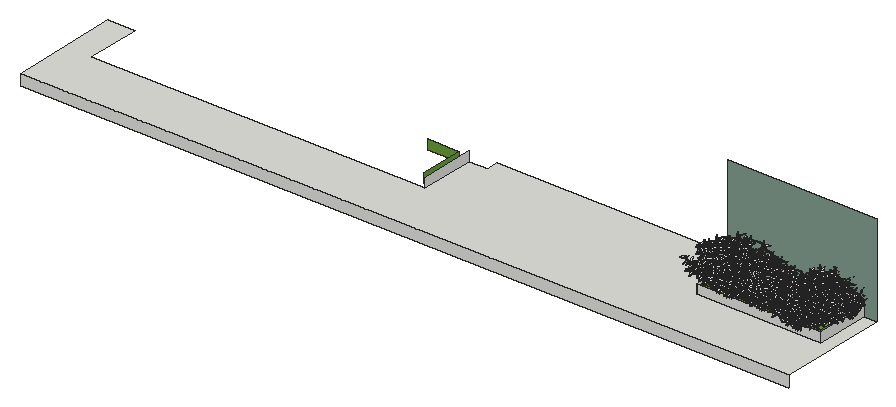
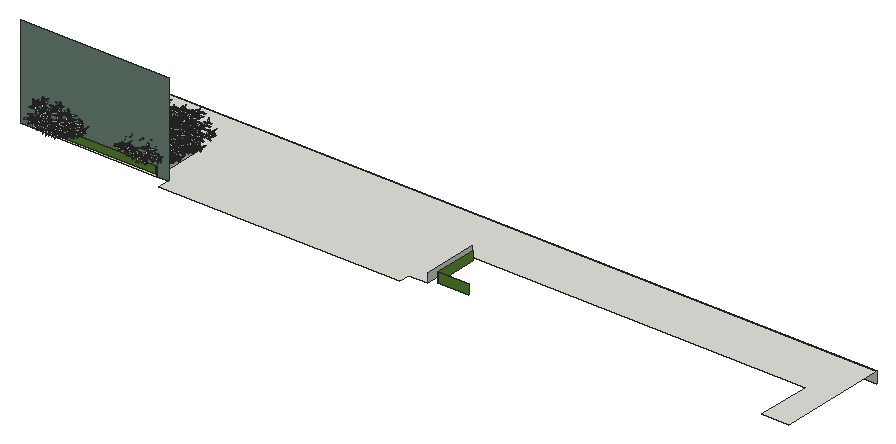
# SketchUp Ruby script. Lengths in inches.
U = 1.inch
M = Sketchup.active_model
def pt(a) = Geom::Point3d.new(a.map { |v| v * U })
def face(e, loops, mat)
  f = e.add_face(loops[0].map { |a| pt(a) })
  loops[1..].each { |l| e.add_face(l.map { |a| pt(a) }).erase! }
  f.material = f.back_material = mat if mat
  f
end
# faces: each face lists its corners as indices into pts; further lists are holes
def faces(e, pts, list, mat = nil) = list.each { |f| face(e, (f[0].is_a?(Array) ? f : [f]).map { |l| l.map { |i| pts[i] } }, mat) }
# xy, xz, yz: faces in a plane at the given z, y or x. An outline is a flat list of corners, or four numbers for a rectangle; further outlines are holes
def ring(l) = l.size == 4 ? [[l[0], l[1]], [l[2], l[1]], [l[2], l[3]], [l[0], l[3]]] : l.each_slice(2).to_a
def flat(e, list, mat, &to3) = list.each { |f| face(e, (f[0].is_a?(Array) ? f : [f]).map { |l| ring(l).map { |u, v| to3.(u, v) } }, mat) }
def xy(e, z, list, mat = nil) = flat(e, list, mat) { |x, y| [x, y, z] }
def xz(e, y, list, mat = nil) = flat(e, list, mat) { |x, z| [x, y, z] }
def yz(e, x, list, mat = nil) = flat(e, list, mat) { |y, z| [x, y, z] }
def lines(e, pts, list) = list.each { |a, b| e.add_line(pt(pts[a]), pt(pts[b])) }
# prism: a flat outline (further loops are holes) pulled along v
def prism(e, loops, v, mat = nil)
  f = face(e, loops, mat); d = Geom::Vector3d.new(v.map { |x| x * U })
  f.pushpull(f.normal.samedirection?(d) ? d.length : -d.length)
end
def box(e, o, s, mat = nil) = prism(e, [[o, [o[0] + s[0], o[1], o[2]], [o[0] + s[0], o[1] + s[1], o[2]], [o[0], o[1] + s[1], o[2]]]], [0, 0, s[2]], mat)
def at(x, y, z, deg = 0) = Geom::Transformation.translation(pt([x, y, z])) * Geom::Transformation.rotation(ORIGIN, Z_AXIS, deg.degrees)
def axes(o, x, y, z) = Geom::Transformation.new([*x, 0, *y, 0, *z, 0, *pt(o).to_a, 1])
def part(name) = M.definitions.add(name)
# library, detail: a bought-in or finely detailed component or shape, given as its bounding box
def library(name, o, s) = part(name).tap { |d| box(d.entities, o, s) }
def detail(e, o, s) = box(e.add_group.entities, o, s)
def put(e, d, t, mat = nil) = e.add_instance(d, t).tap { |i| i.material = mat if mat }
def group(e, t, mat = nil) = e.add_group.tap { |g| g.transformation = t; g.material = mat if mat }.entities
root = M.entities
M.materials.add("[Color H08]").color = [130, 158, 143]
M.materials.add("[Grass Dark Green]").color = [106, 157, 55]
c1 = part("Plane.003")
p = [[-13.75,10.1875,13.53],[-8.85,45.75,19.16],[-0.05,76.91,20.56],[0.09,-0.03,-0.02],[7.48,49.37,17.16],[14.16,9.16,9.9]]
faces(c1.entities,p,[[0,1,2,3],[4,5,3,2]])
c2 = part("spirea_leaf")
put(c2.entities,c1,at(0,0,0))
c3 = part("Plane.002")
p = [[-2.92,82.99,124.67],[-2.92,-0.79,0],[2.92,-0.79,0],[2.92,82.99,124.67],[2.92,149.28,292.15],[-2.92,149.28,292.15],
  [2.92,182.43,464.87],[-2.92,182.43,464.87]]
faces(c3.entities,p,[[0,1,2,3],[3,4,5,0],[5,4,6],[5,6,7]])
c4 = part("spirea_stem")
put(c4.entities,c3,at(0,0,0))
c5 = part("spirea_single")
put(c5.entities,c2,axes([61.07,82.24,152.17],[-0.04534,0.68195,-0.35141],[-0.74248,-0.12758,-0.15177],[-0.19302,0.33055,0.66639]))
put(c5.entities,c2,axes([59.72,73.38,127.91],[0.28617,0.56014,-0.10586],[-0.56688,0.26713,-0.11894],[-0.06012,0.14744,0.61766]))
put(c5.entities,c4,axes([60.19,1.84,0],[0.3441,0,0],[0,0.62,0],[0,0,0.62]))
put(c5.entities,c2,axes([59.67,34.88,53.33],[0.45126,0.21625,-0.53161],[-0.52806,0.42133,-0.27684],[0.2248,0.55563,0.41684]))
put(c5.entities,c2,axes([59.72,42.6,61.76],[0.43966,-0.56732,0.27467],[0.6265,0.43009,-0.11449],[-0.0692,0.28942,0.70855]))
put(c5.entities,c2,axes([60.64,103.19,225.26],[-0.35027,-0.4893,-0.00056],[0.48916,-0.35019,0.01365],[-0.01142,0.00749,0.60159]))
put(c5.entities,c2,axes([59.49,100.02,211.41],[0.59184,-0.32302,0],[0.323,0.59181,-0.00668],[0.0032,0.00586,0.67422]))
put(c5.entities,c2,axes([60.71,98.4,200.52],[0.37279,0.59177,-0.19096],[-0.61923,0.37358,-0.05117],[0.05663,0.18942,0.69752]))
put(c5.entities,c2,axes([60.46,79.17,144.19],[-0.69777,0.02304,-0.21354],[-0.09001,-0.69041,0.21963],[-0.195,0.23624,0.6627]))
put(c5.entities,c2,axes([59.53,75.43,133.01],[0.51977,-0.50179,-0.10513],[0.47164,0.52669,-0.18209],[0.201,0.06172,0.69914]))
put(c5.entities,c2,axes([61.85,65.23,103.75],[-0.33765,-0.67856,0.12705],[0.68306,-0.34887,-0.04799],[0.10005,0.09184,0.75641]))
put(c5.entities,c2,axes([59.93,92.9,176.87],[0.03118,-0.56709,0.29033],[0.62588,0.08155,0.09208],[-0.11899,0.28038,0.56044]))
put(c5.entities,c2,axes([60.8125,96.09,190.88],[-0.43546,0.45576,-0.27755],[-0.47188,-0.49616,-0.07437],[-0.24915,0.14314,0.62595]))
put(c5.entities,c2,axes([61.06,86.21,159.17],[0.68151,0.1886,0.10384],[-0.14294,0.65414,-0.24995],[-0.161,0.21757,0.66147]))
put(c5.entities,c2,axes([61.02,103.72,233.5],[0.15025,0.6695,-0.05975],[-0.66771,0.14162,-0.09212],[-0.07726,0.07802,0.67994]))
put(c5.entities,c2,axes([59.84,60.39,94.71],[0.69689,-0.19053,-0.10513],[0.16077,0.68848,-0.18209],[0.14666,0.15067,0.69914]))
put(c5.entities,c2,axes([60.35,111.25,265.8],[-0.44527,0.00464,-0.00041],[-0.00465,-0.44516,0.0101],[-0.00031,0.0101,0.44518]))
put(c5.entities,c2,axes([62.04,106.17,241.79],[0.58725,0,0],[0,0.58493,-0.0522],[0,0.0522,0.58493]))
put(c5.entities,c2,axes([61.05,108.11,252.87],[-0.04027,-0.58443,0.33381],[0.6723,-0.01918,0.04751],[-0.03168,0.33568,0.58389]))
c6 = part("spirea_noflower")
put(c6.entities,c4,axes([7.4375,15.95,0.02],[-0.05138,-0.02266,0],[0.04001,-0.09072,0.02017],[-0.00814,0.01846,0.09915]))
put(c6.entities,c2,axes([10.92,7.8,33.61],[0.09808,-0.04627,-0.02956],[0.03942,0.10146,-0.02804],[0.03822,0.0141,0.10476]))
put(c6.entities,c2,axes([10.66,8.28,28.22],[-0.09096,-0.06939,0.02274],[0.06684,-0.09374,-0.01869],[0.0294,-0.00154,0.11286]))
put(c6.entities,c2,axes([10.82,7.9375,40.67],[0.02156,-0.10964,0.01223],[0.11005,0.02051,-0.01012],[0.00764,0.01391,0.11128]))
put(c6.entities,c2,axes([10.02,10.22,17.07],[-0.11498,-0.02115,-0.02301],[0.02282,-0.11675,-0.00672],[-0.02136,-0.01089,0.11671]))
put(c6.entities,c2,axes([10.95,7.79,39.34],[0.02073,0.09465,-0.01601],[-0.09582,0.01943,-0.00921],[-0.00571,0.01757,0.09645]))
put(c6.entities,c2,axes([9.92,9.65,18.67],[0.00496,0.12531,-0.00176],[-0.12388,0.00463,-0.01903],[-0.01894,0.00249,0.12396]))
put(c6.entities,c2,axes([11.03,7.9,31.26],[-0.04507,0.08957,0.02798],[-0.0894,-0.05041,0.01738],[0.0285,-0.01651,0.09875]))
put(c6.entities,c2,axes([8.95,12.73,9.62],[-0.04645,-0.07719,-0.07798],[0.10968,-0.03512,-0.03057],[-0.00318,-0.0837,0.08474]))
put(c6.entities,c2,axes([10.44,9.32,22.8],[-0.00519,-0.10396,0.0013],[0.10345,-0.00529,-0.01033],[0.01038,0.00077,0.10358]))
put(c6.entities,c2,axes([9.33,11.85,11.22],[-0.10587,0.06223,0.02547],[-0.06429,-0.1076,-0.00432],[0.01971,-0.0167,0.12273]))
put(c6.entities,c2,axes([10.09,9.85,19.95],[0.08489,-0.07402,0.03033],[0.07003,0.09014,0.02399],[-0.03866,0.00075,0.11004]))
put(c6.entities,c2,axes([10.96,7.75,35.23],[-0.01497,-0.11683,-0.01129],[0.11725,-0.0154,0.00397],[-0.00539,-0.01068,0.11771]))
put(c6.entities,c2,axes([11.1,7.92,37.02],[-0.10922,0.00829,-0.01051],[-0.00995,-0.10807,0.01819],[-0.00895,0.019,0.10801]))
put(c6.entities,c2,axes([10.5,8.65,26.97],[0.0554,-0.10726,-0.03401],[0.10463,0.06305,-0.02842],[0.0414,-0.01582,0.11733]))
put(c6.entities,c2,axes([10.49,8.91,25.59],[0.10848,0.03623,-0.0334],[-0.034,0.11349,0.01266],[0.03566,-0.002,0.11367]))
put(c6.entities,c2,axes([10.54,9.18,23.68],[-0.10862,0.03606,-0.03314],[-0.03404,-0.11355,-0.01198],[-0.03521,-0.00146,0.11382]))
put(c6.entities,c2,axes([10.72,7.76,42.08],[-0.08769,-0.03868,0],[0.03843,-0.08714,0.01068],[-0.00431,0.00977,0.09524]))
put(c6.entities,c2,axes([10.85,7.87,43.91],[-0.03609,0.09811,0.03437],[-0.10225,-0.04006,0.00697],[0.01873,-0.02965,0.1043]))
put(c6.entities,c2,axes([10.98,7.84,46.08],[0.06679,0.02863,0.00008],[-0.02817,0.06574,-0.01287],[-0.00515,0.01179,0.07152]))
put(c6.entities,c2,axes([10.8,7.97,48.125],[-0.06893,0.0419,0.00009],[-0.04141,-0.06814,0.0122],[0.00642,0.01038,0.07974]))
put(c6.entities,c2,axes([10.94,7.82,49.1],[0.01894,-0.07016,0.00008],[0.05795,0.01569,0.04095],[-0.03956,-0.0106,0.06003]))
c7 = part("Spirea")
put(c7.entities,c5,axes([20.99,29.53,3.1875],[0.01954,-0.091,-0.02329],[0.08848,0.02778,-0.02423],[0.03497,-0.01946,0.07433]))
put(c7.entities,c5,axes([16.1875,23.97,1.65],[0.09656,0,0],[0,0.09656,0],[0,0,0.08111]))
put(c7.entities,c6,axes([35.43,25.1,-1.16],[-0.42763,0.26514,-0.05489],[-0.21558,-0.25326,0.32187],[0.16762,0.35071,0.27393]))
put(c7.entities,c6,axes([22.85,19.9,0.53],[0.4898,0.21094,-0.05818],[-0.15904,0.4504,0.20754],[0.15492,-0.20455,0.39699]))
put(c7.entities,c6,axes([25.64,17.62,5.32],[0.39778,0.28453,-0.05716],[-0.26298,0.39808,0.10688],[0.12818,-0.06625,0.39667]))
put(c7.entities,c6,axes([31.05,18.22,-1.16],[0.07698,0.49724,-0.05489],[-0.31736,0.09949,0.32187],[0.38833,-0.01726,0.27393]))
put(c7.entities,c5,axes([20.99,26.3,1.41],[0.06978,-0.07324,-0.00678],[0.06848,0.06856,-0.02532],[0.02721,0.01528,0.08112]))
put(c7.entities,c5,axes([22.49,26.46,1.43],[0.0904,0.01,-0.0061],[-0.01173,0.08633,-0.02277],[0.0039,0.02779,0.07293]))
put(c7.entities,c6,axes([30.45,32.2,-0.81],[0.02285,-0.56892,-0.06212],[0.15135,-0.06541,0.46198],[-0.55338,-0.04138,0.12379]))
put(c7.entities,c6,axes([21.91,22.81,-0.85],[-0.02216,0.50268,-0.05489],[-0.17773,0.05355,0.39666],[0.47473,0.04352,0.14594]))
put(c7.entities,c5,axes([30.1,30.77,0.36],[-0.1011,-0.04459,0],[0.04369,-0.09907,0.0185],[-0.00889,0.02016,0.09095]))
put(c7.entities,c5,axes([21.74,22.85,1.41],[0.07373,0.06926,-0.00678],[-0.06808,0.06896,-0.02532],[-0.01509,0.02732,0.08112]))
put(c7.entities,c5,axes([16.43,23,1.65],[0.06407,0.07017,0],[-0.07017,0.06407,0],[0,0,0.07982]))
put(c7.entities,c5,axes([17.07,18.375,1.34],[0.03932,0.08211,-0.00611],[-0.07957,0.0357,-0.02279],[-0.02155,0.01801,0.073]))
put(c7.entities,c5,axes([28.5,22.43,1.65],[-0.08829,0.05201,0],[-0.05201,-0.08829,0],[0,0,0.08608]))
put(c7.entities,c6,axes([28.93,29.38,-2.32],[-0.56896,-0.02186,-0.06212],[-0.04199,-0.37401,0.36423],[-0.06468,0.43508,0.30998]))
put(c7.entities,c5,axes([30.22,28.68,0.43],[-0.09325,-0.03922,-0.00678],[0.04003,-0.09171,-0.01417],[-0.00078,-0.01869,0.08379]))
put(c7.entities,c5,axes([22.83,20.65,3.32],[-0.01797,0.0853,0],[-0.08403,-0.01771,-0.01259],[-0.01466,-0.00309,0.07213]))
put(c7.entities,c6,axes([24.5,33.17,-1.16],[-0.36679,-0.34444,-0.05489],[0.18883,-0.27379,0.32187],[-0.29538,0.25268,0.27393]))
put(c7.entities,c6,axes([16.17,23.58,-0.85],[0.44167,0.24105,-0.05489],[-0.0301,0.18317,0.39666],[0.24793,-0.40717,0.14594]))
put(c7.entities,c6,axes([15.32,23.08,-1.16],[0.43965,-0.24471,-0.05489],[0.20342,0.26314,0.32187],[-0.15091,-0.35822,0.27393]))
put(c7.entities,c6,axes([25.22,18.48,-2.32],[0.43489,0.36751,-0.06212],[-0.19718,0.32058,0.36423],[0.31883,-0.30303,0.30998]))
put(c7.entities,c6,axes([17.47,17.85,-1.16],[0.50022,0.05434,-0.05489],[0.01396,0.3323,0.32187],[0.08384,-0.37956,0.27393]))
put(c7.entities,c6,axes([19.68,35.94,-1.16],[-0.12258,-0.488,-0.05489],[0.30682,-0.12838,0.32187],[-0.38507,0.05305,0.27393]))
put(c7.entities,c5,axes([20.21,32.32,1.65],[0.059,-0.08211,0],[0.08211,0.059,0],[0,0,0.08493]))
put(c7.entities,c5,axes([30.73,22.42,1.41],[-0.10081,0.00845,-0.00678],[-0.00569,-0.09674,-0.02532],[-0.01021,-0.02949,0.08112]))
put(c7.entities,c6,axes([19.68,37.38,0.39],[-0.15639,-0.58365,0],[0.58365,-0.15639,0],[0,0,0.50756]))
put(c7.entities,c6,axes([14.16,35.57,1.53],[-0.16219,-0.57166,-0.08263],[0.57944,-0.1644,0],[-0.02685,-0.09464,0.49914]))
put(c7.entities,c6,axes([17.58,28.45,-2.32],[0.19381,-0.53538,-0.06212],[0.36907,0.07371,0.36423],[-0.39482,-0.1939,0.30998]))
xy(root,9,[[0,0,600,0,600,85.1875,590.375,85.1875,590.375,43.3125,493.5625,43.3125,493.5625,85.1875,484.36,85.1875,484.36,94.1875,296.4375,94.1875,296.4375,85.1875,281.76,85.1875,281.76,42.875,21.01,42.875,21.01,85.1875,0,85.1875],[[493.5625,43.3125,590.375,85.1875],[495.57,45.32,588.37,83.18]]])
xy(root,9,[[495.57,45.32,588.37,83.18]],"[Grass Dark Green]")
xz(root,0,[[0,0,600,9]])
xz(root,43.3125,[[493.5625,9,590.375,16.375]])
xz(root,45.32,[[495.57,9,588.37,16.375]],"[Grass Dark Green]")
xz(root,80.93,[[253.1,9,277.5,16.375]],"[Grass Dark Green]")
xz(root,83.18,[[495.57,9,588.37,16.375]],"[Grass Dark Green]")
xz(root,85.1875,[[484.36,9,493.5625,9,493.5625,16.375,590.375,16.375,590.375,9,600,9,600,81,484.36,81]],"[Color H08]")
yz(root,277.5,[[47.13,9,80.93,16.375]],"[Grass Dark Green]")
yz(root,281.76,[[42.875,9,85.1875,16.375]])
yz(root,493.5625,[[43.3125,9,85.1875,16.375]])
yz(root,495.57,[[45.32,9,83.18,16.375]],"[Grass Dark Green]")
yz(root,588.37,[[45.32,9,83.18,16.375]],"[Grass Dark Green]")
yz(root,590.375,[[43.3125,9,85.1875,16.375]])
put(root,c7,at(476.89,33.6,13.18))
put(root,c7,at(481.85,47.88,10.65))
put(root,c7,at(488.52,33.6,10.73))
put(root,c7,at(503.7,33.6,13.18))
put(root,c7,at(516.5625,30.28,13.18))
put(root,c7,at(545.375,30.28,13.18))
put(root,c7,at(545.78,28.92,10.41))
put(root,c7,at(546.22,55.15,9.75))
put(root,c7,at(553.9375,37.4,13.18))
